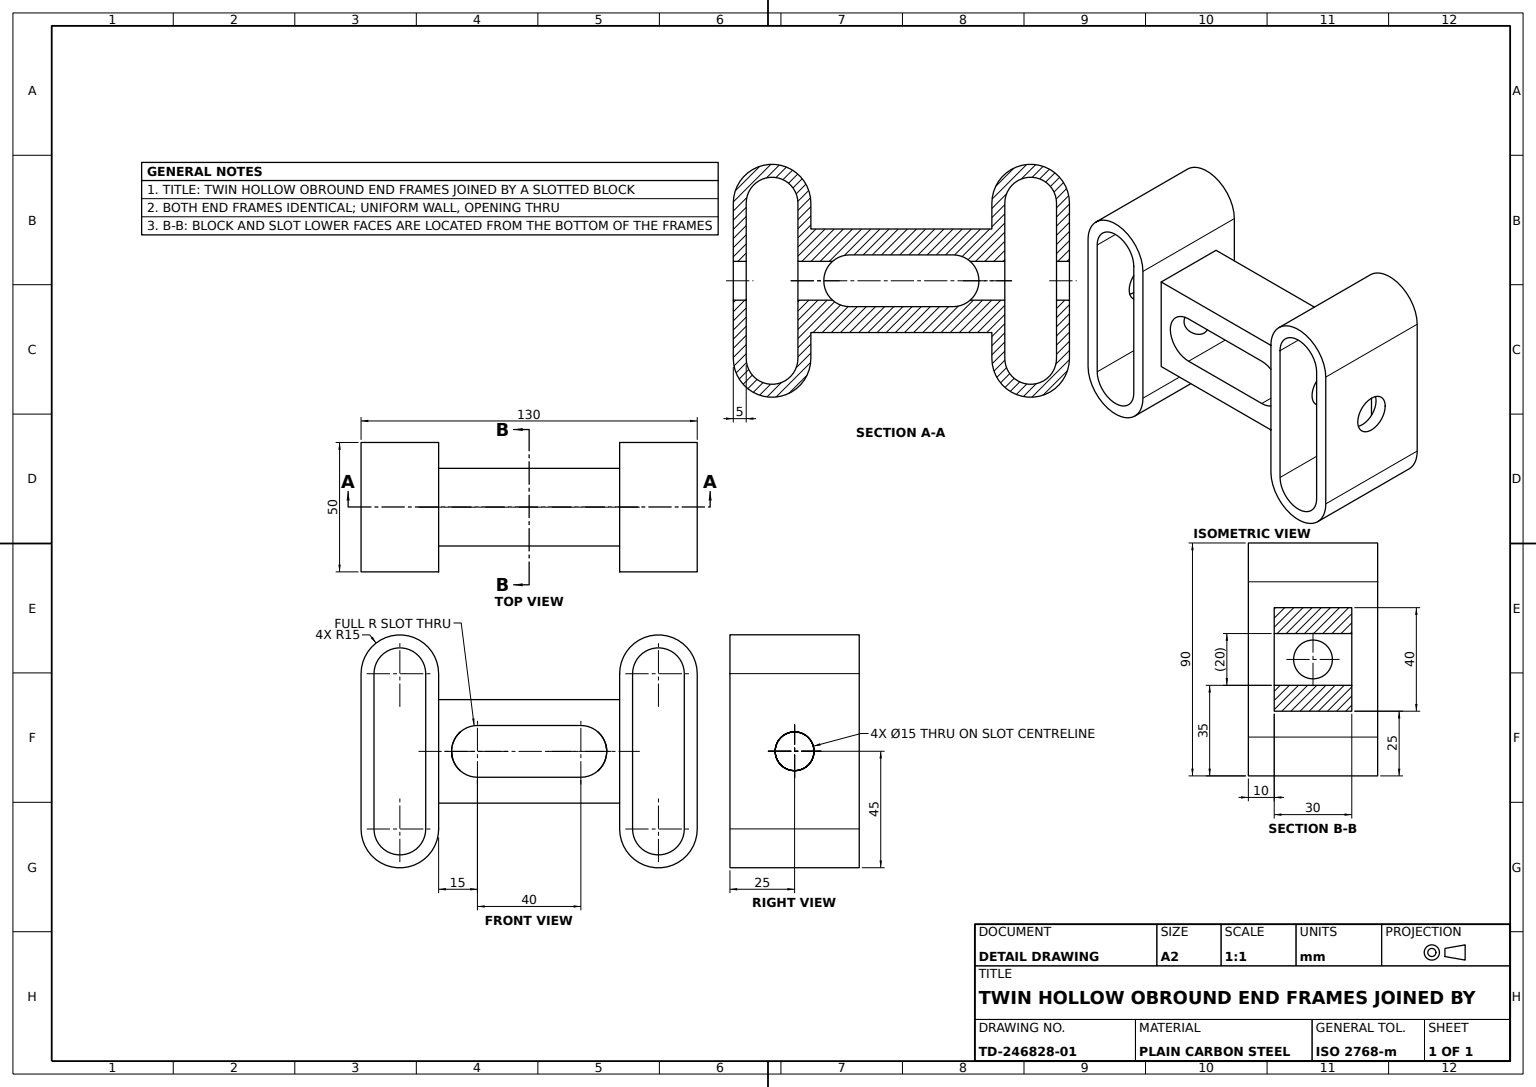
ISO-10303-21;
HEADER;
FILE_DESCRIPTION((''),'2;1');
FILE_NAME('','',(''),(''),'','','');
FILE_SCHEMA(('AUTOMOTIVE_DESIGN'));
ENDSEC;
DATA;
#1=APPLICATION_CONTEXT('');
#2=PRODUCT_CONTEXT('',#1,'mechanical');
#3=PRODUCT('','','',(#2));
#4=PRODUCT_DEFINITION_FORMATION('','',#3);
#5=PRODUCT_DEFINITION_CONTEXT('',#1,'design');
#6=PRODUCT_DEFINITION('','',#4,#5);
#7=PRODUCT_DEFINITION_SHAPE('','',#6);
#8=(LENGTH_UNIT()NAMED_UNIT(*)SI_UNIT(.MILLI.,.METRE.));
#9=(NAMED_UNIT(*)PLANE_ANGLE_UNIT()SI_UNIT($,.RADIAN.));
#10=(NAMED_UNIT(*)SI_UNIT($,.STERADIAN.)SOLID_ANGLE_UNIT());
#11=UNCERTAINTY_MEASURE_WITH_UNIT(LENGTH_MEASURE(1.E-05),#8,'distance_accuracy_value','');
#12=(GEOMETRIC_REPRESENTATION_CONTEXT(3)GLOBAL_UNCERTAINTY_ASSIGNED_CONTEXT((#11))GLOBAL_UNIT_ASSIGNED_CONTEXT((#8,#9,#10))REPRESENTATION_CONTEXT('',''));
#13=CARTESIAN_POINT('',(-65.,30.,40.));
#14=VERTEX_POINT('',#13);
#15=CARTESIAN_POINT('',(-65.,-30.,40.));
#16=VERTEX_POINT('',#15);
#17=DIRECTION('',(0.,-1.,0.));
#18=VECTOR('',#17,1000.);
#19=LINE('',#13,#18);
#20=EDGE_CURVE('',#14,#16,#19,.T.);
#21=ORIENTED_EDGE('',*,*,#20,.T.);
#22=CARTESIAN_POINT('',(-35.,-30.,40.));
#23=VERTEX_POINT('',#22);
#24=CARTESIAN_POINT('',(-50.,-30.,40.));
#25=DIRECTION('',(0.,0.,1.));
#26=DIRECTION('',(-1.,0.,0.));
#27=AXIS2_PLACEMENT_3D('',#24,#25,#26);
#28=CIRCLE('',#27,15.);
#29=EDGE_CURVE('',#16,#23,#28,.T.);
#30=ORIENTED_EDGE('',*,*,#29,.T.);
#31=CARTESIAN_POINT('',(-35.,30.,40.));
#32=VERTEX_POINT('',#31);
#33=DIRECTION('',(0.,1.,0.));
#34=VECTOR('',#33,1000.);
#35=LINE('',#31,#34);
#36=EDGE_CURVE('',#23,#32,#35,.T.);
#37=ORIENTED_EDGE('',*,*,#36,.T.);
#38=CARTESIAN_POINT('',(-50.,30.,40.));
#39=AXIS2_PLACEMENT_3D('',#38,#25,#26);
#40=CIRCLE('',#39,15.);
#41=EDGE_CURVE('',#32,#14,#40,.T.);
#42=ORIENTED_EDGE('',*,*,#41,.T.);
#43=EDGE_LOOP('',(#21,#30,#37,#42));
#44=FACE_OUTER_BOUND('',#43,.T.);
#45=CARTESIAN_POINT('',(-40.,30.,40.));
#46=VERTEX_POINT('',#45);
#47=CARTESIAN_POINT('',(-60.,30.,40.));
#48=VERTEX_POINT('',#47);
#49=CIRCLE('',#39,10.);
#50=EDGE_CURVE('',#46,#48,#49,.T.);
#51=ORIENTED_EDGE('',*,*,#50,.F.);
#52=CARTESIAN_POINT('',(-40.,-30.,40.));
#53=VERTEX_POINT('',#52);
#54=LINE('',#45,#34);
#55=EDGE_CURVE('',#53,#46,#54,.T.);
#56=ORIENTED_EDGE('',*,*,#55,.F.);
#57=CARTESIAN_POINT('',(-60.,-30.,40.));
#58=VERTEX_POINT('',#57);
#59=CIRCLE('',#27,10.);
#60=EDGE_CURVE('',#58,#53,#59,.T.);
#61=ORIENTED_EDGE('',*,*,#60,.F.);
#62=LINE('',#47,#18);
#63=EDGE_CURVE('',#48,#58,#62,.T.);
#64=ORIENTED_EDGE('',*,*,#63,.F.);
#65=EDGE_LOOP('',(#51,#56,#61,#64));
#66=FACE_BOUND('',#65,.T.);
#67=DIRECTION('',(0.,0.,-1.));
#68=AXIS2_PLACEMENT_3D('',#38,#67,#26);
#69=PLANE('',#68);
#70=ADVANCED_FACE('',(#44,#66),#69,.F.);
#71=CARTESIAN_POINT('',(20.,-10.,0.));
#72=VERTEX_POINT('',#71);
#73=CARTESIAN_POINT('',(20.,10.,0.));
#74=VERTEX_POINT('',#73);
#75=CARTESIAN_POINT('',(20.,0.,0.));
#76=DIRECTION('',(1.,0.,0.));
#77=AXIS2_PLACEMENT_3D('',#75,#25,#76);
#78=CIRCLE('',#77,10.);
#79=EDGE_CURVE('',#72,#74,#78,.T.);
#80=ORIENTED_EDGE('',*,*,#79,.F.);
#81=CARTESIAN_POINT('',(20.,-10.,30.));
#82=VERTEX_POINT('',#81);
#83=VECTOR('',#67,1000.);
#84=LINE('',#81,#83);
#85=EDGE_CURVE('',#82,#72,#84,.T.);
#86=ORIENTED_EDGE('',*,*,#85,.F.);
#87=CARTESIAN_POINT('',(20.,10.,30.));
#88=VERTEX_POINT('',#87);
#89=CARTESIAN_POINT('',(20.,0.,30.));
#90=AXIS2_PLACEMENT_3D('',#89,#25,#76);
#91=CIRCLE('',#90,10.);
#92=EDGE_CURVE('',#82,#88,#91,.T.);
#93=ORIENTED_EDGE('',*,*,#92,.T.);
#94=LINE('',#87,#83);
#95=EDGE_CURVE('',#88,#74,#94,.T.);
#96=ORIENTED_EDGE('',*,*,#95,.T.);
#97=EDGE_LOOP('',(#80,#86,#93,#96));
#98=FACE_OUTER_BOUND('',#97,.T.);
#99=CARTESIAN_POINT('',(30.,0.,22.5));
#100=VERTEX_POINT('',#99);
#101=CARTESIAN_POINT('',(30.,0.,7.5));
#102=VERTEX_POINT('',#101);
#103=CARTESIAN_POINT('',(30.,0.256348,22.5));
#104=CARTESIAN_POINT('',(29.989997,0.51597,22.486678));
#105=CARTESIAN_POINT('',(29.950223,1.029232,22.433522));
#106=CARTESIAN_POINT('',(29.920725,1.281515,22.394051));
#107=CARTESIAN_POINT('',(29.84389,1.777891,22.290636));
#108=CARTESIAN_POINT('',(29.796548,2.021982,22.226688));
#109=CARTESIAN_POINT('',(29.68502,2.502232,22.074763));
#110=CARTESIAN_POINT('',(29.620556,2.738926,21.986394));
#111=CARTESIAN_POINT('',(29.408431,3.421795,21.69231));
#112=CARTESIAN_POINT('',(29.241051,3.846586,21.456536));
#113=CARTESIAN_POINT('',(28.867875,4.642632,20.91008));
#114=CARTESIAN_POINT('',(28.665435,5.006227,20.604281));
#115=CARTESIAN_POINT('',(28.353308,5.500933,20.103411));
#116=CARTESIAN_POINT('',(28.247655,5.657705,19.929068));
#117=CARTESIAN_POINT('',(28.035266,5.955497,19.5648));
#118=CARTESIAN_POINT('',(27.928409,6.096585,19.374572));
#119=CARTESIAN_POINT('',(27.615685,6.489485,18.789132));
#120=CARTESIAN_POINT('',(27.415376,6.714116,18.376421));
#121=CARTESIAN_POINT('',(27.147088,6.995421,17.715046));
#122=CARTESIAN_POINT('',(27.063104,7.079822,17.487453));
#123=CARTESIAN_POINT('',(26.910911,7.22846,17.015111));
#124=CARTESIAN_POINT('',(26.84332,7.292095,16.771604));
#125=CARTESIAN_POINT('',(26.732665,7.394383,16.279193));
#126=CARTESIAN_POINT('',(26.689123,7.43352,16.028839));
#127=CARTESIAN_POINT('',(26.62986,7.486424,15.518834));
#128=CARTESIAN_POINT('',(26.61434,7.500034,15.257114));
#129=CARTESIAN_POINT('',(26.614417,7.499966,14.740908));
#130=CARTESIAN_POINT('',(26.629605,7.486647,14.484964));
#131=CARTESIAN_POINT('',(26.688242,7.43431,13.977167));
#132=CARTESIAN_POINT('',(26.73197,7.395022,13.724069));
#133=CARTESIAN_POINT('',(26.899297,7.240357,12.978958));
#134=CARTESIAN_POINT('',(27.054895,7.091995,12.512754));
#135=CARTESIAN_POINT('',(27.3248,6.809133,11.846605));
#136=CARTESIAN_POINT('',(27.421492,6.704056,11.629166));
#137=CARTESIAN_POINT('',(27.621041,6.476315,11.209982));
#138=CARTESIAN_POINT('',(27.723681,6.353948,11.008482));
#139=CARTESIAN_POINT('',(28.03551,5.961725,10.42536));
#140=CARTESIAN_POINT('',(28.248484,5.667069,10.064803));
#141=CARTESIAN_POINT('',(28.561725,5.170605,9.562142));
#142=CARTESIAN_POINT('',(28.665639,4.994991,9.40031));
#143=CARTESIAN_POINT('',(28.86576,4.6305,9.095346));
#144=CARTESIAN_POINT('',(28.962237,4.441323,8.951744));
#145=CARTESIAN_POINT('',(29.238455,3.852159,8.54726));
#146=CARTESIAN_POINT('',(29.405137,3.430839,8.312312));
#147=CARTESIAN_POINT('',(29.617919,2.748172,8.017235));
#148=CARTESIAN_POINT('',(29.682804,2.51081,7.92827));
#149=CARTESIAN_POINT('',(29.794823,2.030343,7.775649));
#150=CARTESIAN_POINT('',(29.842431,1.786014,7.711334));
#151=CARTESIAN_POINT('',(29.919783,1.288871,7.607212));
#152=CARTESIAN_POINT('',(29.949533,1.03606,7.567402));
#153=CARTESIAN_POINT('',(29.989733,0.521403,7.513674));
#154=CARTESIAN_POINT('',(30.,0.259573,7.5));
#155=B_SPLINE_CURVE_WITH_KNOTS('',3,(#99,#103,#104,#105,#106,#107,#108,#109,#110,#111,#112,#113,#114,#115,#116,#117,#118,#119,#120,#121,#122,#123,#124,#125,#126,#127,#128,#129,#130,#131,#132,#133,#134,#135,#136,#137,#138,#139,#140,#141,#142,#143,#144,#145,#146,#147,#148,#149,#150,#151,#152,#153,#154,#101),.UNSPECIFIED.,.F.,.F.,(4,2,2,2,2,2,2,2,2,2,2,2,2,2,2,2,2,2,2,2,2,2,2,2,2,2,4),(0.024564477,0.02533051,0.026096543,0.026862577,0.02762861,0.029160677,0.030692744,0.031458777,0.03222481,0.033756877,0.03452291,0.035288944,0.036054977,0.03682101,0.037587044,0.038353077,0.039885144,0.040651177,0.041417211,0.042949277,0.043715311,0.044481344,0.046013411,0.046779444,0.047545477,0.048311511,0.049077544),.UNSPECIFIED.);
#156=EDGE_CURVE('',#100,#102,#155,.T.);
#157=ORIENTED_EDGE('',*,*,#156,.F.);
#158=CARTESIAN_POINT('',(30.,-0.520235,7.5));
#159=CARTESIAN_POINT('',(29.959688,-1.028227,7.553514));
#160=CARTESIAN_POINT('',(29.844714,-1.77335,7.708253));
#161=CARTESIAN_POINT('',(29.796987,-2.02,7.772715));
#162=CARTESIAN_POINT('',(29.684959,-2.502583,7.925318));
#163=CARTESIAN_POINT('',(29.621281,-2.736302,8.012611));
#164=CARTESIAN_POINT('',(29.480549,-3.18992,8.207698));
#165=CARTESIAN_POINT('',(29.403488,-3.409814,8.315498));
#166=CARTESIAN_POINT('',(29.237585,-3.836592,8.550972));
#167=CARTESIAN_POINT('',(29.148278,-4.044405,8.679326));
#168=CARTESIAN_POINT('',(28.868804,-4.64081,9.088537));
#169=CARTESIAN_POINT('',(28.667494,-5.00276,9.392508));
#170=CARTESIAN_POINT('',(28.250162,-5.664617,10.062016));
#171=CARTESIAN_POINT('',(28.033355,-5.964614,10.429135));
#172=CARTESIAN_POINT('',(27.617757,-6.487001,11.206817));
#173=CARTESIAN_POINT('',(27.416893,-6.71252,11.61987));
#174=CARTESIAN_POINT('',(27.146477,-6.996065,12.286445));
#175=CARTESIAN_POINT('',(27.061248,-7.081665,12.517876));
#176=CARTESIAN_POINT('',(26.909788,-7.229525,12.988811));
#177=CARTESIAN_POINT('',(26.843143,-7.29226,13.229125));
#178=CARTESIAN_POINT('',(26.732675,-7.394372,13.720819));
#179=CARTESIAN_POINT('',(26.688795,-7.433815,13.972744));
#180=CARTESIAN_POINT('',(26.629306,-7.486915,14.487188));
#181=CARTESIAN_POINT('',(26.614382,-7.499997,14.743832));
#182=CARTESIAN_POINT('',(26.614375,-7.500003,15.255975));
#183=CARTESIAN_POINT('',(26.629289,-7.486927,15.511474));
#184=CARTESIAN_POINT('',(26.687976,-7.43455,16.021346));
#185=CARTESIAN_POINT('',(26.732132,-7.39487,16.276532));
#186=CARTESIAN_POINT('',(26.843016,-7.292382,16.770539));
#187=CARTESIAN_POINT('',(26.909847,-7.229469,17.0114));
#188=CARTESIAN_POINT('',(27.061377,-7.081537,17.482496));
#189=CARTESIAN_POINT('',(27.146576,-6.995971,17.713853));
#190=CARTESIAN_POINT('',(27.417743,-6.71161,18.382115));
#191=CARTESIAN_POINT('',(27.619082,-6.48548,18.795869));
#192=CARTESIAN_POINT('',(28.035382,-5.96192,19.574449));
#193=CARTESIAN_POINT('',(28.252518,-5.661163,19.941891));
#194=CARTESIAN_POINT('',(28.669262,-4.999671,20.6102));
#195=CARTESIAN_POINT('',(28.869784,-4.638691,20.912894));
#196=CARTESIAN_POINT('',(29.24023,-3.848205,21.455315));
#197=CARTESIAN_POINT('',(29.410854,-3.414904,21.695701));
#198=CARTESIAN_POINT('',(29.62189,-2.734166,21.988228));
#199=CARTESIAN_POINT('',(29.685274,-2.501183,22.075109));
#200=CARTESIAN_POINT('',(29.796482,-2.022222,22.226597));
#201=CARTESIAN_POINT('',(29.844534,-1.77473,22.291506));
#202=CARTESIAN_POINT('',(29.960638,-1.021641,22.447762));
#203=CARTESIAN_POINT('',(30.,-0.513772,22.5));
#204=B_SPLINE_CURVE_WITH_KNOTS('',3,(#101,#158,#159,#160,#161,#162,#163,#164,#165,#166,#167,#168,#169,#170,#171,#172,#173,#174,#175,#176,#177,#178,#179,#180,#181,#182,#183,#184,#185,#186,#187,#188,#189,#190,#191,#192,#193,#194,#195,#196,#197,#198,#199,#200,#201,#202,#203,#99),.UNSPECIFIED.,.F.,.F.,(4,2,2,2,2,2,2,2,2,2,2,2,2,2,2,2,2,2,2,2,2,2,2,4),(0.,0.00153528,0.00230292,0.00307056,0.003838199,0.004605839,0.006141119,0.007676399,0.009211679,0.009979319,0.010746959,0.011514598,0.012282238,0.013049878,0.013817518,0.014585158,0.015352798,0.016888078,0.018423358,0.019958637,0.021493917,0.022261557,0.023029197,0.024564477),.UNSPECIFIED.);
#205=EDGE_CURVE('',#102,#100,#204,.T.);
#206=ORIENTED_EDGE('',*,*,#205,.F.);
#207=EDGE_LOOP('',(#157,#206));
#208=FACE_BOUND('',#207,.T.);
#209=AXIS2_PLACEMENT_3D('',#89,#67,#26);
#210=CYLINDRICAL_SURFACE('',#209,10.);
#211=ADVANCED_FACE('',(#98,#208),#210,.F.);
#212=CARTESIAN_POINT('',(-30.,0.,0.));
#213=VERTEX_POINT('',#212);
#214=CARTESIAN_POINT('',(-20.,-10.,0.));
#215=VERTEX_POINT('',#214);
#216=CARTESIAN_POINT('',(-20.,0.,0.));
#217=AXIS2_PLACEMENT_3D('',#216,#25,#76);
#218=CIRCLE('',#217,10.);
#219=EDGE_CURVE('',#213,#215,#218,.T.);
#220=ORIENTED_EDGE('',*,*,#219,.F.);
#221=CARTESIAN_POINT('',(-30.,0.,7.5));
#222=VERTEX_POINT('',#221);
#223=CARTESIAN_POINT('',(-30.,0.,30.));
#224=LINE('',#223,#83);
#225=EDGE_CURVE('',#222,#213,#224,.T.);
#226=ORIENTED_EDGE('',*,*,#225,.F.);
#227=CARTESIAN_POINT('',(-30.,0.,22.5));
#228=VERTEX_POINT('',#227);
#229=CARTESIAN_POINT('',(-30.,-0.256348,22.5));
#230=CARTESIAN_POINT('',(-29.989997,-0.51597,22.486678));
#231=CARTESIAN_POINT('',(-29.950223,-1.029232,22.433522));
#232=CARTESIAN_POINT('',(-29.920725,-1.281515,22.394051));
#233=CARTESIAN_POINT('',(-29.84389,-1.777891,22.290636));
#234=CARTESIAN_POINT('',(-29.796548,-2.021982,22.226688));
#235=CARTESIAN_POINT('',(-29.68502,-2.502232,22.074763));
#236=CARTESIAN_POINT('',(-29.620556,-2.738926,21.986394));
#237=CARTESIAN_POINT('',(-29.408431,-3.421795,21.69231));
#238=CARTESIAN_POINT('',(-29.241051,-3.846586,21.456536));
#239=CARTESIAN_POINT('',(-28.867875,-4.642632,20.91008));
#240=CARTESIAN_POINT('',(-28.665435,-5.006227,20.604281));
#241=CARTESIAN_POINT('',(-28.353308,-5.500933,20.103411));
#242=CARTESIAN_POINT('',(-28.247655,-5.657705,19.929068));
#243=CARTESIAN_POINT('',(-28.035266,-5.955497,19.5648));
#244=CARTESIAN_POINT('',(-27.928409,-6.096585,19.374572));
#245=CARTESIAN_POINT('',(-27.615685,-6.489485,18.789132));
#246=CARTESIAN_POINT('',(-27.415376,-6.714116,18.376421));
#247=CARTESIAN_POINT('',(-27.147088,-6.995421,17.715046));
#248=CARTESIAN_POINT('',(-27.063104,-7.079822,17.487453));
#249=CARTESIAN_POINT('',(-26.910911,-7.22846,17.015111));
#250=CARTESIAN_POINT('',(-26.84332,-7.292095,16.771604));
#251=CARTESIAN_POINT('',(-26.732665,-7.394383,16.279193));
#252=CARTESIAN_POINT('',(-26.689123,-7.43352,16.028839));
#253=CARTESIAN_POINT('',(-26.62986,-7.486424,15.518834));
#254=CARTESIAN_POINT('',(-26.61434,-7.500034,15.257114));
#255=CARTESIAN_POINT('',(-26.614417,-7.499966,14.740908));
#256=CARTESIAN_POINT('',(-26.629605,-7.486647,14.484964));
#257=CARTESIAN_POINT('',(-26.688242,-7.43431,13.977167));
#258=CARTESIAN_POINT('',(-26.73197,-7.395022,13.724069));
#259=CARTESIAN_POINT('',(-26.899297,-7.240357,12.978958));
#260=CARTESIAN_POINT('',(-27.054895,-7.091995,12.512754));
#261=CARTESIAN_POINT('',(-27.3248,-6.809133,11.846605));
#262=CARTESIAN_POINT('',(-27.421492,-6.704056,11.629166));
#263=CARTESIAN_POINT('',(-27.621041,-6.476315,11.209982));
#264=CARTESIAN_POINT('',(-27.723681,-6.353948,11.008482));
#265=CARTESIAN_POINT('',(-28.03551,-5.961725,10.42536));
#266=CARTESIAN_POINT('',(-28.248484,-5.667069,10.064803));
#267=CARTESIAN_POINT('',(-28.561725,-5.170605,9.562142));
#268=CARTESIAN_POINT('',(-28.665639,-4.994991,9.40031));
#269=CARTESIAN_POINT('',(-28.86576,-4.6305,9.095346));
#270=CARTESIAN_POINT('',(-28.962237,-4.441323,8.951744));
#271=CARTESIAN_POINT('',(-29.238455,-3.852159,8.54726));
#272=CARTESIAN_POINT('',(-29.405137,-3.430839,8.312312));
#273=CARTESIAN_POINT('',(-29.617919,-2.748172,8.017235));
#274=CARTESIAN_POINT('',(-29.682804,-2.51081,7.92827));
#275=CARTESIAN_POINT('',(-29.794823,-2.030343,7.775649));
#276=CARTESIAN_POINT('',(-29.842431,-1.786014,7.711334));
#277=CARTESIAN_POINT('',(-29.919783,-1.288871,7.607212));
#278=CARTESIAN_POINT('',(-29.949533,-1.03606,7.567402));
#279=CARTESIAN_POINT('',(-29.989733,-0.521403,7.513674));
#280=CARTESIAN_POINT('',(-30.,-0.259573,7.5));
#281=B_SPLINE_CURVE_WITH_KNOTS('',3,(#227,#229,#230,#231,#232,#233,#234,#235,#236,#237,#238,#239,#240,#241,#242,#243,#244,#245,#246,#247,#248,#249,#250,#251,#252,#253,#254,#255,#256,#257,#258,#259,#260,#261,#262,#263,#264,#265,#266,#267,#268,#269,#270,#271,#272,#273,#274,#275,#276,#277,#278,#279,#280,#221),.UNSPECIFIED.,.F.,.F.,(4,2,2,2,2,2,2,2,2,2,2,2,2,2,2,2,2,2,2,2,2,2,2,2,2,2,4),(0.024564477,0.02533051,0.026096543,0.026862577,0.02762861,0.029160677,0.030692744,0.031458777,0.03222481,0.033756877,0.03452291,0.035288944,0.036054977,0.03682101,0.037587044,0.038353077,0.039885144,0.040651177,0.041417211,0.042949277,0.043715311,0.044481344,0.046013411,0.046779444,0.047545477,0.048311511,0.049077544),.UNSPECIFIED.);
#282=EDGE_CURVE('',#228,#222,#281,.T.);
#283=ORIENTED_EDGE('',*,*,#282,.F.);
#284=VERTEX_POINT('',#223);
#285=EDGE_CURVE('',#284,#228,#224,.T.);
#286=ORIENTED_EDGE('',*,*,#285,.F.);
#287=CARTESIAN_POINT('',(-20.,-10.,30.));
#288=VERTEX_POINT('',#287);
#289=CARTESIAN_POINT('',(-20.,0.,30.));
#290=AXIS2_PLACEMENT_3D('',#289,#25,#76);
#291=CIRCLE('',#290,10.);
#292=EDGE_CURVE('',#284,#288,#291,.T.);
#293=ORIENTED_EDGE('',*,*,#292,.T.);
#294=LINE('',#287,#83);
#295=EDGE_CURVE('',#288,#215,#294,.T.);
#296=ORIENTED_EDGE('',*,*,#295,.T.);
#297=EDGE_LOOP('',(#220,#226,#283,#286,#293,#296));
#298=FACE_OUTER_BOUND('',#297,.T.);
#299=AXIS2_PLACEMENT_3D('',#289,#67,#26);
#300=CYLINDRICAL_SURFACE('',#299,10.);
#301=ADVANCED_FACE('',(#298),#300,.F.);
#302=ORIENTED_EDGE('',*,*,#205,.T.);
#303=CARTESIAN_POINT('',(40.,0.,22.5));
#304=VERTEX_POINT('',#303);
#305=CARTESIAN_POINT('',(-95.,0.,22.5));
#306=VECTOR('',#76,1000.);
#307=LINE('',#305,#306);
#308=EDGE_CURVE('',#100,#304,#307,.T.);
#309=ORIENTED_EDGE('',*,*,#308,.T.);
#310=CARTESIAN_POINT('',(40.,0.,7.5));
#311=VERTEX_POINT('',#310);
#312=CARTESIAN_POINT('',(40.,0.,15.));
#313=AXIS2_PLACEMENT_3D('',#312,#76,#33);
#314=CIRCLE('',#313,7.5);
#315=EDGE_CURVE('',#304,#311,#314,.T.);
#316=ORIENTED_EDGE('',*,*,#315,.T.);
#317=CARTESIAN_POINT('',(-95.,0.,7.5));
#318=LINE('',#317,#306);
#319=EDGE_CURVE('',#102,#311,#318,.T.);
#320=ORIENTED_EDGE('',*,*,#319,.F.);
#321=EDGE_LOOP('',(#302,#309,#316,#320));
#322=FACE_OUTER_BOUND('',#321,.T.);
#323=CARTESIAN_POINT('',(-95.,0.,15.));
#324=AXIS2_PLACEMENT_3D('',#323,#76,#67);
#325=CYLINDRICAL_SURFACE('',#324,7.5);
#326=ADVANCED_FACE('',(#322),#325,.F.);
#327=CARTESIAN_POINT('',(65.,0.,22.5));
#328=VERTEX_POINT('',#327);
#329=CARTESIAN_POINT('',(65.,0.,7.5));
#330=VERTEX_POINT('',#329);
#331=CARTESIAN_POINT('',(65.,0.,15.));
#332=AXIS2_PLACEMENT_3D('',#331,#26,#25);
#333=CIRCLE('',#332,7.5);
#334=EDGE_CURVE('',#328,#330,#333,.T.);
#335=ORIENTED_EDGE('',*,*,#334,.F.);
#336=CARTESIAN_POINT('',(60.,0.,22.5));
#337=VERTEX_POINT('',#336);
#338=EDGE_CURVE('',#337,#328,#307,.T.);
#339=ORIENTED_EDGE('',*,*,#338,.F.);
#340=CARTESIAN_POINT('',(60.,0.,7.5));
#341=VERTEX_POINT('',#340);
#342=CARTESIAN_POINT('',(60.,0.,15.));
#343=AXIS2_PLACEMENT_3D('',#342,#26,#17);
#344=CIRCLE('',#343,7.5);
#345=EDGE_CURVE('',#337,#341,#344,.T.);
#346=ORIENTED_EDGE('',*,*,#345,.T.);
#347=EDGE_CURVE('',#341,#330,#318,.T.);
#348=ORIENTED_EDGE('',*,*,#347,.T.);
#349=EDGE_LOOP('',(#335,#339,#346,#348));
#350=FACE_OUTER_BOUND('',#349,.T.);
#351=ADVANCED_FACE('',(#350),#325,.F.);
#352=ORIENTED_EDGE('',*,*,#50,.T.);
#353=CARTESIAN_POINT('',(-60.,30.,-10.));
#354=VERTEX_POINT('',#353);
#355=LINE('',#47,#83);
#356=EDGE_CURVE('',#48,#354,#355,.T.);
#357=ORIENTED_EDGE('',*,*,#356,.T.);
#358=CARTESIAN_POINT('',(-40.,30.,-10.));
#359=VERTEX_POINT('',#358);
#360=CARTESIAN_POINT('',(-50.,30.,-10.));
#361=AXIS2_PLACEMENT_3D('',#360,#25,#26);
#362=CIRCLE('',#361,10.);
#363=EDGE_CURVE('',#359,#354,#362,.T.);
#364=ORIENTED_EDGE('',*,*,#363,.F.);
#365=LINE('',#45,#83);
#366=EDGE_CURVE('',#46,#359,#365,.T.);
#367=ORIENTED_EDGE('',*,*,#366,.F.);
#368=EDGE_LOOP('',(#352,#357,#364,#367));
#369=FACE_OUTER_BOUND('',#368,.T.);
#370=CYLINDRICAL_SURFACE('',#68,10.);
#371=ADVANCED_FACE('',(#369),#370,.F.);
#372=CARTESIAN_POINT('',(-20.,10.,0.));
#373=VERTEX_POINT('',#372);
#374=VECTOR('',#26,1000.);
#375=LINE('',#73,#374);
#376=EDGE_CURVE('',#74,#373,#375,.T.);
#377=ORIENTED_EDGE('',*,*,#376,.T.);
#378=EDGE_CURVE('',#373,#213,#218,.T.);
#379=ORIENTED_EDGE('',*,*,#378,.T.);
#380=ORIENTED_EDGE('',*,*,#219,.T.);
#381=LINE('',#71,#306);
#382=EDGE_CURVE('',#215,#72,#381,.T.);
#383=ORIENTED_EDGE('',*,*,#382,.T.);
#384=ORIENTED_EDGE('',*,*,#79,.T.);
#385=EDGE_LOOP('',(#377,#379,#380,#383,#384));
#386=FACE_BOUND('',#385,.T.);
#387=CARTESIAN_POINT('',(-35.,-20.,0.));
#388=VERTEX_POINT('',#387);
#389=CARTESIAN_POINT('',(35.,-20.,0.));
#390=VERTEX_POINT('',#389);
#391=LINE('',#387,#306);
#392=EDGE_CURVE('',#388,#390,#391,.T.);
#393=ORIENTED_EDGE('',*,*,#392,.F.);
#394=CARTESIAN_POINT('',(-35.,20.,0.));
#395=VERTEX_POINT('',#394);
#396=LINE('',#394,#18);
#397=EDGE_CURVE('',#395,#388,#396,.T.);
#398=ORIENTED_EDGE('',*,*,#397,.F.);
#399=CARTESIAN_POINT('',(35.,20.,0.));
#400=VERTEX_POINT('',#399);
#401=LINE('',#394,#374);
#402=EDGE_CURVE('',#400,#395,#401,.T.);
#403=ORIENTED_EDGE('',*,*,#402,.F.);
#404=LINE('',#399,#34);
#405=EDGE_CURVE('',#390,#400,#404,.T.);
#406=ORIENTED_EDGE('',*,*,#405,.F.);
#407=EDGE_LOOP('',(#393,#398,#403,#406));
#408=FACE_OUTER_BOUND('',#407,.T.);
#409=CARTESIAN_POINT('',(0.,0.,0.));
#410=AXIS2_PLACEMENT_3D('',#409,#67,#26);
#411=PLANE('',#410);
#412=ADVANCED_FACE('',(#386,#408),#411,.T.);
#413=CARTESIAN_POINT('',(35.,-30.,40.));
#414=VERTEX_POINT('',#413);
#415=CARTESIAN_POINT('',(35.,-30.,-10.));
#416=VERTEX_POINT('',#415);
#417=LINE('',#413,#83);
#418=EDGE_CURVE('',#414,#416,#417,.T.);
#419=ORIENTED_EDGE('',*,*,#418,.T.);
#420=CARTESIAN_POINT('',(65.,-30.,-10.));
#421=VERTEX_POINT('',#420);
#422=CARTESIAN_POINT('',(50.,-30.,-10.));
#423=AXIS2_PLACEMENT_3D('',#422,#25,#76);
#424=CIRCLE('',#423,15.);
#425=EDGE_CURVE('',#416,#421,#424,.T.);
#426=ORIENTED_EDGE('',*,*,#425,.T.);
#427=CARTESIAN_POINT('',(65.,-30.,40.));
#428=VERTEX_POINT('',#427);
#429=LINE('',#427,#83);
#430=EDGE_CURVE('',#428,#421,#429,.T.);
#431=ORIENTED_EDGE('',*,*,#430,.F.);
#432=CARTESIAN_POINT('',(50.,-30.,40.));
#433=AXIS2_PLACEMENT_3D('',#432,#25,#76);
#434=CIRCLE('',#433,15.);
#435=EDGE_CURVE('',#414,#428,#434,.T.);
#436=ORIENTED_EDGE('',*,*,#435,.F.);
#437=EDGE_LOOP('',(#419,#426,#431,#436));
#438=FACE_OUTER_BOUND('',#437,.T.);
#439=AXIS2_PLACEMENT_3D('',#432,#67,#26);
#440=CYLINDRICAL_SURFACE('',#439,15.);
#441=ADVANCED_FACE('',(#438),#440,.T.);
#442=CARTESIAN_POINT('',(35.,30.,-10.));
#443=VERTEX_POINT('',#442);
#444=LINE('',#442,#18);
#445=EDGE_CURVE('',#443,#416,#444,.T.);
#446=ORIENTED_EDGE('',*,*,#445,.T.);
#447=ORIENTED_EDGE('',*,*,#418,.F.);
#448=CARTESIAN_POINT('',(35.,30.,40.));
#449=VERTEX_POINT('',#448);
#450=LINE('',#448,#18);
#451=EDGE_CURVE('',#449,#414,#450,.T.);
#452=ORIENTED_EDGE('',*,*,#451,.F.);
#453=LINE('',#448,#83);
#454=EDGE_CURVE('',#449,#443,#453,.T.);
#455=ORIENTED_EDGE('',*,*,#454,.T.);
#456=EDGE_LOOP('',(#446,#447,#452,#455));
#457=FACE_OUTER_BOUND('',#456,.T.);
#458=CARTESIAN_POINT('',(35.,20.,30.));
#459=VERTEX_POINT('',#458);
#460=LINE('',#458,#83);
#461=EDGE_CURVE('',#459,#400,#460,.T.);
#462=ORIENTED_EDGE('',*,*,#461,.F.);
#463=CARTESIAN_POINT('',(35.,-20.,30.));
#464=VERTEX_POINT('',#463);
#465=LINE('',#458,#34);
#466=EDGE_CURVE('',#464,#459,#465,.T.);
#467=ORIENTED_EDGE('',*,*,#466,.F.);
#468=LINE('',#463,#83);
#469=EDGE_CURVE('',#464,#390,#468,.T.);
#470=ORIENTED_EDGE('',*,*,#469,.T.);
#471=ORIENTED_EDGE('',*,*,#405,.T.);
#472=EDGE_LOOP('',(#462,#467,#470,#471));
#473=FACE_BOUND('',#472,.T.);
#474=AXIS2_PLACEMENT_3D('',#448,#76,#67);
#475=PLANE('',#474);
#476=ADVANCED_FACE('',(#457,#473),#475,.F.);
#477=CARTESIAN_POINT('',(-60.,0.,22.5));
#478=VERTEX_POINT('',#477);
#479=CARTESIAN_POINT('',(-60.,0.,7.5));
#480=VERTEX_POINT('',#479);
#481=CARTESIAN_POINT('',(-60.,0.,15.));
#482=AXIS2_PLACEMENT_3D('',#481,#76,#33);
#483=CIRCLE('',#482,7.5);
#484=EDGE_CURVE('',#478,#480,#483,.T.);
#485=ORIENTED_EDGE('',*,*,#484,.T.);
#486=CARTESIAN_POINT('',(-65.,0.,7.5));
#487=VERTEX_POINT('',#486);
#488=EDGE_CURVE('',#487,#480,#318,.T.);
#489=ORIENTED_EDGE('',*,*,#488,.F.);
#490=CARTESIAN_POINT('',(-65.,0.,22.5));
#491=VERTEX_POINT('',#490);
#492=CARTESIAN_POINT('',(-65.,0.,15.));
#493=AXIS2_PLACEMENT_3D('',#492,#76,#67);
#494=CIRCLE('',#493,7.5);
#495=EDGE_CURVE('',#491,#487,#494,.T.);
#496=ORIENTED_EDGE('',*,*,#495,.F.);
#497=EDGE_CURVE('',#491,#478,#307,.T.);
#498=ORIENTED_EDGE('',*,*,#497,.T.);
#499=EDGE_LOOP('',(#485,#489,#496,#498));
#500=FACE_OUTER_BOUND('',#499,.T.);
#501=ADVANCED_FACE('',(#500),#325,.F.);
#502=CARTESIAN_POINT('',(-35.,30.,-10.));
#503=VERTEX_POINT('',#502);
#504=CARTESIAN_POINT('',(-65.,30.,-10.));
#505=VERTEX_POINT('',#504);
#506=CIRCLE('',#361,15.);
#507=EDGE_CURVE('',#503,#505,#506,.T.);
#508=ORIENTED_EDGE('',*,*,#507,.T.);
#509=LINE('',#13,#83);
#510=EDGE_CURVE('',#14,#505,#509,.T.);
#511=ORIENTED_EDGE('',*,*,#510,.F.);
#512=ORIENTED_EDGE('',*,*,#41,.F.);
#513=LINE('',#31,#83);
#514=EDGE_CURVE('',#32,#503,#513,.T.);
#515=ORIENTED_EDGE('',*,*,#514,.T.);
#516=EDGE_LOOP('',(#508,#511,#512,#515));
#517=FACE_OUTER_BOUND('',#516,.T.);
#518=CYLINDRICAL_SURFACE('',#68,15.);
#519=ADVANCED_FACE('',(#517),#518,.T.);
#520=CARTESIAN_POINT('',(-35.,20.,30.));
#521=VERTEX_POINT('',#520);
#522=CARTESIAN_POINT('',(-35.,-20.,30.));
#523=VERTEX_POINT('',#522);
#524=LINE('',#520,#18);
#525=EDGE_CURVE('',#521,#523,#524,.T.);
#526=ORIENTED_EDGE('',*,*,#525,.F.);
#527=LINE('',#520,#83);
#528=EDGE_CURVE('',#521,#395,#527,.T.);
#529=ORIENTED_EDGE('',*,*,#528,.T.);
#530=ORIENTED_EDGE('',*,*,#397,.T.);
#531=LINE('',#522,#83);
#532=EDGE_CURVE('',#523,#388,#531,.T.);
#533=ORIENTED_EDGE('',*,*,#532,.F.);
#534=EDGE_LOOP('',(#526,#529,#530,#533));
#535=FACE_BOUND('',#534,.T.);
#536=CARTESIAN_POINT('',(-35.,-30.,-10.));
#537=VERTEX_POINT('',#536);
#538=LINE('',#22,#83);
#539=EDGE_CURVE('',#23,#537,#538,.T.);
#540=ORIENTED_EDGE('',*,*,#539,.T.);
#541=LINE('',#502,#34);
#542=EDGE_CURVE('',#537,#503,#541,.T.);
#543=ORIENTED_EDGE('',*,*,#542,.T.);
#544=ORIENTED_EDGE('',*,*,#514,.F.);
#545=ORIENTED_EDGE('',*,*,#36,.F.);
#546=EDGE_LOOP('',(#540,#543,#544,#545));
#547=FACE_OUTER_BOUND('',#546,.T.);
#548=AXIS2_PLACEMENT_3D('',#31,#26,#25);
#549=PLANE('',#548);
#550=ADVANCED_FACE('',(#535,#547),#549,.F.);
#551=ORIENTED_EDGE('',*,*,#402,.T.);
#552=ORIENTED_EDGE('',*,*,#528,.F.);
#553=LINE('',#520,#374);
#554=EDGE_CURVE('',#459,#521,#553,.T.);
#555=ORIENTED_EDGE('',*,*,#554,.F.);
#556=ORIENTED_EDGE('',*,*,#461,.T.);
#557=EDGE_LOOP('',(#551,#552,#555,#556));
#558=FACE_OUTER_BOUND('',#557,.T.);
#559=AXIS2_PLACEMENT_3D('',#520,#17,#67);
#560=PLANE('',#559);
#561=ADVANCED_FACE('',(#558),#560,.F.);
#562=CARTESIAN_POINT('',(40.,-30.,40.));
#563=VERTEX_POINT('',#562);
#564=CARTESIAN_POINT('',(60.,-30.,40.));
#565=VERTEX_POINT('',#564);
#566=CIRCLE('',#433,10.);
#567=EDGE_CURVE('',#563,#565,#566,.T.);
#568=ORIENTED_EDGE('',*,*,#567,.T.);
#569=CARTESIAN_POINT('',(60.,-30.,-10.));
#570=VERTEX_POINT('',#569);
#571=LINE('',#564,#83);
#572=EDGE_CURVE('',#565,#570,#571,.T.);
#573=ORIENTED_EDGE('',*,*,#572,.T.);
#574=CARTESIAN_POINT('',(40.,-30.,-10.));
#575=VERTEX_POINT('',#574);
#576=CIRCLE('',#423,10.);
#577=EDGE_CURVE('',#575,#570,#576,.T.);
#578=ORIENTED_EDGE('',*,*,#577,.F.);
#579=LINE('',#562,#83);
#580=EDGE_CURVE('',#563,#575,#579,.T.);
#581=ORIENTED_EDGE('',*,*,#580,.F.);
#582=EDGE_LOOP('',(#568,#573,#578,#581));
#583=FACE_OUTER_BOUND('',#582,.T.);
#584=CYLINDRICAL_SURFACE('',#439,10.);
#585=ADVANCED_FACE('',(#583),#584,.F.);
#586=EDGE_CURVE('',#480,#478,#483,.T.);
#587=ORIENTED_EDGE('',*,*,#586,.F.);
#588=ORIENTED_EDGE('',*,*,#484,.F.);
#589=EDGE_LOOP('',(#587,#588));
#590=FACE_BOUND('',#589,.T.);
#591=CARTESIAN_POINT('',(-60.,-30.,-10.));
#592=VERTEX_POINT('',#591);
#593=LINE('',#353,#18);
#594=EDGE_CURVE('',#354,#592,#593,.T.);
#595=ORIENTED_EDGE('',*,*,#594,.F.);
#596=ORIENTED_EDGE('',*,*,#356,.F.);
#597=ORIENTED_EDGE('',*,*,#63,.T.);
#598=LINE('',#57,#83);
#599=EDGE_CURVE('',#58,#592,#598,.T.);
#600=ORIENTED_EDGE('',*,*,#599,.T.);
#601=EDGE_LOOP('',(#595,#596,#597,#600));
#602=FACE_OUTER_BOUND('',#601,.T.);
#603=AXIS2_PLACEMENT_3D('',#47,#76,#33);
#604=PLANE('',#603);
#605=ADVANCED_FACE('',(#590,#602),#604,.T.);
#606=CARTESIAN_POINT('',(-65.,-30.,-10.));
#607=VERTEX_POINT('',#606);
#608=LINE('',#15,#83);
#609=EDGE_CURVE('',#16,#607,#608,.T.);
#610=ORIENTED_EDGE('',*,*,#609,.T.);
#611=CARTESIAN_POINT('',(-50.,-30.,-10.));
#612=AXIS2_PLACEMENT_3D('',#611,#25,#26);
#613=CIRCLE('',#612,15.);
#614=EDGE_CURVE('',#607,#537,#613,.T.);
#615=ORIENTED_EDGE('',*,*,#614,.T.);
#616=ORIENTED_EDGE('',*,*,#539,.F.);
#617=ORIENTED_EDGE('',*,*,#29,.F.);
#618=EDGE_LOOP('',(#610,#615,#616,#617));
#619=FACE_OUTER_BOUND('',#618,.T.);
#620=AXIS2_PLACEMENT_3D('',#24,#67,#26);
#621=CYLINDRICAL_SURFACE('',#620,15.);
#622=ADVANCED_FACE('',(#619),#621,.T.);
#623=ORIENTED_EDGE('',*,*,#507,.F.);
#624=ORIENTED_EDGE('',*,*,#542,.F.);
#625=ORIENTED_EDGE('',*,*,#614,.F.);
#626=LINE('',#504,#18);
#627=EDGE_CURVE('',#505,#607,#626,.T.);
#628=ORIENTED_EDGE('',*,*,#627,.F.);
#629=EDGE_LOOP('',(#623,#624,#625,#628));
#630=FACE_OUTER_BOUND('',#629,.T.);
#631=CARTESIAN_POINT('',(-40.,-30.,-10.));
#632=VERTEX_POINT('',#631);
#633=LINE('',#358,#34);
#634=EDGE_CURVE('',#632,#359,#633,.T.);
#635=ORIENTED_EDGE('',*,*,#634,.T.);
#636=ORIENTED_EDGE('',*,*,#363,.T.);
#637=ORIENTED_EDGE('',*,*,#594,.T.);
#638=CIRCLE('',#612,10.);
#639=EDGE_CURVE('',#592,#632,#638,.T.);
#640=ORIENTED_EDGE('',*,*,#639,.T.);
#641=EDGE_LOOP('',(#635,#636,#637,#640));
#642=FACE_BOUND('',#641,.T.);
#643=AXIS2_PLACEMENT_3D('',#360,#67,#26);
#644=PLANE('',#643);
#645=ADVANCED_FACE('',(#630,#642),#644,.T.);
#646=CARTESIAN_POINT('',(65.,30.,-10.));
#647=VERTEX_POINT('',#646);
#648=CARTESIAN_POINT('',(50.,30.,-10.));
#649=AXIS2_PLACEMENT_3D('',#648,#25,#76);
#650=CIRCLE('',#649,15.);
#651=EDGE_CURVE('',#647,#443,#650,.T.);
#652=ORIENTED_EDGE('',*,*,#651,.F.);
#653=LINE('',#646,#34);
#654=EDGE_CURVE('',#421,#647,#653,.T.);
#655=ORIENTED_EDGE('',*,*,#654,.F.);
#656=ORIENTED_EDGE('',*,*,#425,.F.);
#657=ORIENTED_EDGE('',*,*,#445,.F.);
#658=EDGE_LOOP('',(#652,#655,#656,#657));
#659=FACE_OUTER_BOUND('',#658,.T.);
#660=CARTESIAN_POINT('',(60.,30.,-10.));
#661=VERTEX_POINT('',#660);
#662=LINE('',#660,#34);
#663=EDGE_CURVE('',#570,#661,#662,.T.);
#664=ORIENTED_EDGE('',*,*,#663,.T.);
#665=CARTESIAN_POINT('',(40.,30.,-10.));
#666=VERTEX_POINT('',#665);
#667=CIRCLE('',#649,10.);
#668=EDGE_CURVE('',#661,#666,#667,.T.);
#669=ORIENTED_EDGE('',*,*,#668,.T.);
#670=LINE('',#665,#18);
#671=EDGE_CURVE('',#666,#575,#670,.T.);
#672=ORIENTED_EDGE('',*,*,#671,.T.);
#673=ORIENTED_EDGE('',*,*,#577,.T.);
#674=EDGE_LOOP('',(#664,#669,#672,#673));
#675=FACE_BOUND('',#674,.T.);
#676=PLANE('',#649);
#677=ADVANCED_FACE('',(#659,#675),#676,.F.);
#678=CARTESIAN_POINT('',(-40.,0.,7.5));
#679=VERTEX_POINT('',#678);
#680=CARTESIAN_POINT('',(-40.,0.,22.5));
#681=VERTEX_POINT('',#680);
#682=CARTESIAN_POINT('',(-40.,0.,15.));
#683=AXIS2_PLACEMENT_3D('',#682,#26,#17);
#684=CIRCLE('',#683,7.5);
#685=EDGE_CURVE('',#679,#681,#684,.T.);
#686=ORIENTED_EDGE('',*,*,#685,.T.);
#687=EDGE_CURVE('',#681,#228,#307,.T.);
#688=ORIENTED_EDGE('',*,*,#687,.T.);
#689=ORIENTED_EDGE('',*,*,#282,.T.);
#690=EDGE_CURVE('',#679,#222,#318,.T.);
#691=ORIENTED_EDGE('',*,*,#690,.F.);
#692=EDGE_LOOP('',(#686,#688,#689,#691));
#693=FACE_OUTER_BOUND('',#692,.T.);
#694=ADVANCED_FACE('',(#693),#325,.F.);
#695=CARTESIAN_POINT('',(65.,30.,40.));
#696=VERTEX_POINT('',#695);
#697=LINE('',#695,#83);
#698=EDGE_CURVE('',#696,#647,#697,.T.);
#699=ORIENTED_EDGE('',*,*,#698,.T.);
#700=ORIENTED_EDGE('',*,*,#651,.T.);
#701=ORIENTED_EDGE('',*,*,#454,.F.);
#702=CARTESIAN_POINT('',(50.,30.,40.));
#703=AXIS2_PLACEMENT_3D('',#702,#25,#76);
#704=CIRCLE('',#703,15.);
#705=EDGE_CURVE('',#696,#449,#704,.T.);
#706=ORIENTED_EDGE('',*,*,#705,.F.);
#707=EDGE_LOOP('',(#699,#700,#701,#706));
#708=FACE_OUTER_BOUND('',#707,.T.);
#709=AXIS2_PLACEMENT_3D('',#702,#67,#26);
#710=CYLINDRICAL_SURFACE('',#709,15.);
#711=ADVANCED_FACE('',(#708),#710,.T.);
#712=EDGE_CURVE('',#681,#679,#684,.T.);
#713=ORIENTED_EDGE('',*,*,#712,.T.);
#714=ORIENTED_EDGE('',*,*,#690,.T.);
#715=CARTESIAN_POINT('',(-30.,0.520235,7.5));
#716=CARTESIAN_POINT('',(-29.959688,1.028227,7.553514));
#717=CARTESIAN_POINT('',(-29.844714,1.77335,7.708253));
#718=CARTESIAN_POINT('',(-29.796987,2.02,7.772715));
#719=CARTESIAN_POINT('',(-29.684959,2.502583,7.925318));
#720=CARTESIAN_POINT('',(-29.621281,2.736302,8.012611));
#721=CARTESIAN_POINT('',(-29.480549,3.18992,8.207698));
#722=CARTESIAN_POINT('',(-29.403488,3.409814,8.315498));
#723=CARTESIAN_POINT('',(-29.237585,3.836592,8.550972));
#724=CARTESIAN_POINT('',(-29.148278,4.044405,8.679326));
#725=CARTESIAN_POINT('',(-28.868804,4.64081,9.088537));
#726=CARTESIAN_POINT('',(-28.667494,5.00276,9.392508));
#727=CARTESIAN_POINT('',(-28.250162,5.664617,10.062016));
#728=CARTESIAN_POINT('',(-28.033355,5.964614,10.429135));
#729=CARTESIAN_POINT('',(-27.617757,6.487001,11.206817));
#730=CARTESIAN_POINT('',(-27.416893,6.71252,11.61987));
#731=CARTESIAN_POINT('',(-27.146477,6.996065,12.286445));
#732=CARTESIAN_POINT('',(-27.061248,7.081665,12.517876));
#733=CARTESIAN_POINT('',(-26.909788,7.229525,12.988811));
#734=CARTESIAN_POINT('',(-26.843143,7.29226,13.229125));
#735=CARTESIAN_POINT('',(-26.732675,7.394372,13.720819));
#736=CARTESIAN_POINT('',(-26.688795,7.433815,13.972744));
#737=CARTESIAN_POINT('',(-26.629306,7.486915,14.487188));
#738=CARTESIAN_POINT('',(-26.614382,7.499997,14.743832));
#739=CARTESIAN_POINT('',(-26.614375,7.500003,15.255975));
#740=CARTESIAN_POINT('',(-26.629289,7.486927,15.511474));
#741=CARTESIAN_POINT('',(-26.687976,7.43455,16.021346));
#742=CARTESIAN_POINT('',(-26.732132,7.39487,16.276532));
#743=CARTESIAN_POINT('',(-26.843016,7.292382,16.770539));
#744=CARTESIAN_POINT('',(-26.909847,7.229469,17.0114));
#745=CARTESIAN_POINT('',(-27.061377,7.081537,17.482496));
#746=CARTESIAN_POINT('',(-27.146576,6.995971,17.713853));
#747=CARTESIAN_POINT('',(-27.417743,6.71161,18.382115));
#748=CARTESIAN_POINT('',(-27.619082,6.48548,18.795869));
#749=CARTESIAN_POINT('',(-28.035382,5.96192,19.574449));
#750=CARTESIAN_POINT('',(-28.252518,5.661163,19.941891));
#751=CARTESIAN_POINT('',(-28.669262,4.999671,20.6102));
#752=CARTESIAN_POINT('',(-28.869784,4.638691,20.912894));
#753=CARTESIAN_POINT('',(-29.24023,3.848205,21.455315));
#754=CARTESIAN_POINT('',(-29.410854,3.414904,21.695701));
#755=CARTESIAN_POINT('',(-29.62189,2.734166,21.988228));
#756=CARTESIAN_POINT('',(-29.685274,2.501183,22.075109));
#757=CARTESIAN_POINT('',(-29.796482,2.022222,22.226597));
#758=CARTESIAN_POINT('',(-29.844534,1.77473,22.291506));
#759=CARTESIAN_POINT('',(-29.960638,1.021641,22.447762));
#760=CARTESIAN_POINT('',(-30.,0.513772,22.5));
#761=B_SPLINE_CURVE_WITH_KNOTS('',3,(#221,#715,#716,#717,#718,#719,#720,#721,#722,#723,#724,#725,#726,#727,#728,#729,#730,#731,#732,#733,#734,#735,#736,#737,#738,#739,#740,#741,#742,#743,#744,#745,#746,#747,#748,#749,#750,#751,#752,#753,#754,#755,#756,#757,#758,#759,#760,#227),.UNSPECIFIED.,.F.,.F.,(4,2,2,2,2,2,2,2,2,2,2,2,2,2,2,2,2,2,2,2,2,2,2,4),(0.,0.00153528,0.00230292,0.00307056,0.003838199,0.004605839,0.006141119,0.007676399,0.009211679,0.009979319,0.010746959,0.011514598,0.012282238,0.013049878,0.013817518,0.014585158,0.015352798,0.016888078,0.018423358,0.019958637,0.021493917,0.022261557,0.023029197,0.024564477),.UNSPECIFIED.);
#762=EDGE_CURVE('',#222,#228,#761,.T.);
#763=ORIENTED_EDGE('',*,*,#762,.T.);
#764=ORIENTED_EDGE('',*,*,#687,.F.);
#765=EDGE_LOOP('',(#713,#714,#763,#764));
#766=FACE_OUTER_BOUND('',#765,.T.);
#767=ADVANCED_FACE('',(#766),#325,.F.);
#768=EDGE_CURVE('',#487,#491,#494,.T.);
#769=ORIENTED_EDGE('',*,*,#768,.F.);
#770=ORIENTED_EDGE('',*,*,#488,.T.);
#771=ORIENTED_EDGE('',*,*,#586,.T.);
#772=ORIENTED_EDGE('',*,*,#497,.F.);
#773=EDGE_LOOP('',(#769,#770,#771,#772));
#774=FACE_OUTER_BOUND('',#773,.T.);
#775=ADVANCED_FACE('',(#774),#325,.F.);
#776=LINE('',#81,#306);
#777=EDGE_CURVE('',#288,#82,#776,.T.);
#778=ORIENTED_EDGE('',*,*,#777,.T.);
#779=ORIENTED_EDGE('',*,*,#85,.T.);
#780=ORIENTED_EDGE('',*,*,#382,.F.);
#781=ORIENTED_EDGE('',*,*,#295,.F.);
#782=EDGE_LOOP('',(#778,#779,#780,#781));
#783=FACE_OUTER_BOUND('',#782,.T.);
#784=AXIS2_PLACEMENT_3D('',#81,#33,#26);
#785=PLANE('',#784);
#786=ADVANCED_FACE('',(#783),#785,.T.);
#787=ORIENTED_EDGE('',*,*,#376,.F.);
#788=ORIENTED_EDGE('',*,*,#95,.F.);
#789=CARTESIAN_POINT('',(-20.,10.,30.));
#790=VERTEX_POINT('',#789);
#791=LINE('',#87,#374);
#792=EDGE_CURVE('',#88,#790,#791,.T.);
#793=ORIENTED_EDGE('',*,*,#792,.T.);
#794=LINE('',#789,#83);
#795=EDGE_CURVE('',#790,#373,#794,.T.);
#796=ORIENTED_EDGE('',*,*,#795,.T.);
#797=EDGE_LOOP('',(#787,#788,#793,#796));
#798=FACE_OUTER_BOUND('',#797,.T.);
#799=AXIS2_PLACEMENT_3D('',#87,#17,#76);
#800=PLANE('',#799);
#801=ADVANCED_FACE('',(#798),#800,.T.);
#802=ORIENTED_EDGE('',*,*,#319,.T.);
#803=EDGE_CURVE('',#311,#304,#314,.T.);
#804=ORIENTED_EDGE('',*,*,#803,.T.);
#805=ORIENTED_EDGE('',*,*,#308,.F.);
#806=ORIENTED_EDGE('',*,*,#156,.T.);
#807=EDGE_LOOP('',(#802,#804,#805,#806));
#808=FACE_OUTER_BOUND('',#807,.T.);
#809=ADVANCED_FACE('',(#808),#325,.F.);
#810=ORIENTED_EDGE('',*,*,#338,.T.);
#811=EDGE_CURVE('',#330,#328,#333,.T.);
#812=ORIENTED_EDGE('',*,*,#811,.F.);
#813=ORIENTED_EDGE('',*,*,#347,.F.);
#814=EDGE_CURVE('',#341,#337,#344,.T.);
#815=ORIENTED_EDGE('',*,*,#814,.T.);
#816=EDGE_LOOP('',(#810,#812,#813,#815));
#817=FACE_OUTER_BOUND('',#816,.T.);
#818=ADVANCED_FACE('',(#817),#325,.F.);
#819=LINE('',#695,#34);
#820=EDGE_CURVE('',#428,#696,#819,.T.);
#821=ORIENTED_EDGE('',*,*,#820,.F.);
#822=ORIENTED_EDGE('',*,*,#430,.T.);
#823=ORIENTED_EDGE('',*,*,#654,.T.);
#824=ORIENTED_EDGE('',*,*,#698,.F.);
#825=EDGE_LOOP('',(#821,#822,#823,#824));
#826=FACE_OUTER_BOUND('',#825,.T.);
#827=ORIENTED_EDGE('',*,*,#334,.T.);
#828=ORIENTED_EDGE('',*,*,#811,.T.);
#829=EDGE_LOOP('',(#827,#828));
#830=FACE_BOUND('',#829,.T.);
#831=AXIS2_PLACEMENT_3D('',#695,#26,#25);
#832=PLANE('',#831);
#833=ADVANCED_FACE('',(#826,#830),#832,.F.);
#834=ORIENTED_EDGE('',*,*,#768,.T.);
#835=ORIENTED_EDGE('',*,*,#495,.T.);
#836=EDGE_LOOP('',(#834,#835));
#837=FACE_BOUND('',#836,.T.);
#838=ORIENTED_EDGE('',*,*,#627,.T.);
#839=ORIENTED_EDGE('',*,*,#609,.F.);
#840=ORIENTED_EDGE('',*,*,#20,.F.);
#841=ORIENTED_EDGE('',*,*,#510,.T.);
#842=EDGE_LOOP('',(#838,#839,#840,#841));
#843=FACE_OUTER_BOUND('',#842,.T.);
#844=AXIS2_PLACEMENT_3D('',#13,#76,#67);
#845=PLANE('',#844);
#846=ADVANCED_FACE('',(#837,#843),#845,.F.);
#847=ORIENTED_EDGE('',*,*,#685,.F.);
#848=ORIENTED_EDGE('',*,*,#712,.F.);
#849=EDGE_LOOP('',(#847,#848));
#850=FACE_BOUND('',#849,.T.);
#851=ORIENTED_EDGE('',*,*,#55,.T.);
#852=ORIENTED_EDGE('',*,*,#366,.T.);
#853=ORIENTED_EDGE('',*,*,#634,.F.);
#854=LINE('',#52,#83);
#855=EDGE_CURVE('',#53,#632,#854,.T.);
#856=ORIENTED_EDGE('',*,*,#855,.F.);
#857=EDGE_LOOP('',(#851,#852,#853,#856));
#858=FACE_OUTER_BOUND('',#857,.T.);
#859=AXIS2_PLACEMENT_3D('',#45,#26,#17);
#860=PLANE('',#859);
#861=ADVANCED_FACE('',(#850,#858),#860,.T.);
#862=ORIENTED_EDGE('',*,*,#572,.F.);
#863=CARTESIAN_POINT('',(60.,30.,40.));
#864=VERTEX_POINT('',#863);
#865=LINE('',#863,#34);
#866=EDGE_CURVE('',#565,#864,#865,.T.);
#867=ORIENTED_EDGE('',*,*,#866,.T.);
#868=LINE('',#863,#83);
#869=EDGE_CURVE('',#864,#661,#868,.T.);
#870=ORIENTED_EDGE('',*,*,#869,.T.);
#871=ORIENTED_EDGE('',*,*,#663,.F.);
#872=EDGE_LOOP('',(#862,#867,#870,#871));
#873=FACE_OUTER_BOUND('',#872,.T.);
#874=ORIENTED_EDGE('',*,*,#345,.F.);
#875=ORIENTED_EDGE('',*,*,#814,.F.);
#876=EDGE_LOOP('',(#874,#875));
#877=FACE_BOUND('',#876,.T.);
#878=AXIS2_PLACEMENT_3D('',#863,#26,#17);
#879=PLANE('',#878);
#880=ADVANCED_FACE('',(#873,#877),#879,.T.);
#881=ORIENTED_EDGE('',*,*,#392,.T.);
#882=ORIENTED_EDGE('',*,*,#469,.F.);
#883=LINE('',#522,#306);
#884=EDGE_CURVE('',#523,#464,#883,.T.);
#885=ORIENTED_EDGE('',*,*,#884,.F.);
#886=ORIENTED_EDGE('',*,*,#532,.T.);
#887=EDGE_LOOP('',(#881,#882,#885,#886));
#888=FACE_OUTER_BOUND('',#887,.T.);
#889=AXIS2_PLACEMENT_3D('',#522,#33,#25);
#890=PLANE('',#889);
#891=ADVANCED_FACE('',(#888),#890,.F.);
#892=EDGE_CURVE('',#790,#284,#291,.T.);
#893=ORIENTED_EDGE('',*,*,#892,.T.);
#894=ORIENTED_EDGE('',*,*,#285,.T.);
#895=ORIENTED_EDGE('',*,*,#762,.F.);
#896=ORIENTED_EDGE('',*,*,#225,.T.);
#897=ORIENTED_EDGE('',*,*,#378,.F.);
#898=ORIENTED_EDGE('',*,*,#795,.F.);
#899=EDGE_LOOP('',(#893,#894,#895,#896,#897,#898));
#900=FACE_OUTER_BOUND('',#899,.T.);
#901=ADVANCED_FACE('',(#900),#300,.F.);
#902=ORIENTED_EDGE('',*,*,#599,.F.);
#903=ORIENTED_EDGE('',*,*,#60,.T.);
#904=ORIENTED_EDGE('',*,*,#855,.T.);
#905=ORIENTED_EDGE('',*,*,#639,.F.);
#906=EDGE_LOOP('',(#902,#903,#904,#905));
#907=FACE_OUTER_BOUND('',#906,.T.);
#908=CYLINDRICAL_SURFACE('',#620,10.);
#909=ADVANCED_FACE('',(#907),#908,.F.);
#910=CARTESIAN_POINT('',(40.,30.,40.));
#911=VERTEX_POINT('',#910);
#912=CIRCLE('',#703,10.);
#913=EDGE_CURVE('',#864,#911,#912,.T.);
#914=ORIENTED_EDGE('',*,*,#913,.T.);
#915=LINE('',#910,#83);
#916=EDGE_CURVE('',#911,#666,#915,.T.);
#917=ORIENTED_EDGE('',*,*,#916,.T.);
#918=ORIENTED_EDGE('',*,*,#668,.F.);
#919=ORIENTED_EDGE('',*,*,#869,.F.);
#920=EDGE_LOOP('',(#914,#917,#918,#919));
#921=FACE_OUTER_BOUND('',#920,.T.);
#922=CYLINDRICAL_SURFACE('',#709,10.);
#923=ADVANCED_FACE('',(#921),#922,.F.);
#924=ORIENTED_EDGE('',*,*,#315,.F.);
#925=ORIENTED_EDGE('',*,*,#803,.F.);
#926=EDGE_LOOP('',(#924,#925));
#927=FACE_BOUND('',#926,.T.);
#928=LINE('',#910,#18);
#929=EDGE_CURVE('',#911,#563,#928,.T.);
#930=ORIENTED_EDGE('',*,*,#929,.T.);
#931=ORIENTED_EDGE('',*,*,#580,.T.);
#932=ORIENTED_EDGE('',*,*,#671,.F.);
#933=ORIENTED_EDGE('',*,*,#916,.F.);
#934=EDGE_LOOP('',(#930,#931,#932,#933));
#935=FACE_OUTER_BOUND('',#934,.T.);
#936=AXIS2_PLACEMENT_3D('',#910,#76,#33);
#937=PLANE('',#936);
#938=ADVANCED_FACE('',(#927,#935),#937,.T.);
#939=ORIENTED_EDGE('',*,*,#92,.F.);
#940=ORIENTED_EDGE('',*,*,#777,.F.);
#941=ORIENTED_EDGE('',*,*,#292,.F.);
#942=ORIENTED_EDGE('',*,*,#892,.F.);
#943=ORIENTED_EDGE('',*,*,#792,.F.);
#944=EDGE_LOOP('',(#939,#940,#941,#942,#943));
#945=FACE_BOUND('',#944,.T.);
#946=ORIENTED_EDGE('',*,*,#554,.T.);
#947=ORIENTED_EDGE('',*,*,#525,.T.);
#948=ORIENTED_EDGE('',*,*,#884,.T.);
#949=ORIENTED_EDGE('',*,*,#466,.T.);
#950=EDGE_LOOP('',(#946,#947,#948,#949));
#951=FACE_OUTER_BOUND('',#950,.T.);
#952=CARTESIAN_POINT('',(0.,0.,30.));
#953=AXIS2_PLACEMENT_3D('',#952,#67,#26);
#954=PLANE('',#953);
#955=ADVANCED_FACE('',(#945,#951),#954,.F.);
#956=ORIENTED_EDGE('',*,*,#705,.T.);
#957=ORIENTED_EDGE('',*,*,#451,.T.);
#958=ORIENTED_EDGE('',*,*,#435,.T.);
#959=ORIENTED_EDGE('',*,*,#820,.T.);
#960=EDGE_LOOP('',(#956,#957,#958,#959));
#961=FACE_OUTER_BOUND('',#960,.T.);
#962=ORIENTED_EDGE('',*,*,#866,.F.);
#963=ORIENTED_EDGE('',*,*,#567,.F.);
#964=ORIENTED_EDGE('',*,*,#929,.F.);
#965=ORIENTED_EDGE('',*,*,#913,.F.);
#966=EDGE_LOOP('',(#962,#963,#964,#965));
#967=FACE_BOUND('',#966,.T.);
#968=PLANE('',#703);
#969=ADVANCED_FACE('',(#961,#967),#968,.T.);
#970=CLOSED_SHELL('',(#70,#211,#301,#326,#351,#371,#412,#441,#476,#501,#519,#550,#561,#585,#605,#622,#645,#677,#694,#711,#767,#775,#786,#801,#809,#818,#833,#846,#861,#880,#891,#901,#909,#923,#938,#955,#969));
#971=MANIFOLD_SOLID_BREP('',#970);
#972=ADVANCED_BREP_SHAPE_REPRESENTATION('',(#971),#12);
#973=SHAPE_DEFINITION_REPRESENTATION(#7,#972);
ENDSEC;
END-ISO-10303-21;
